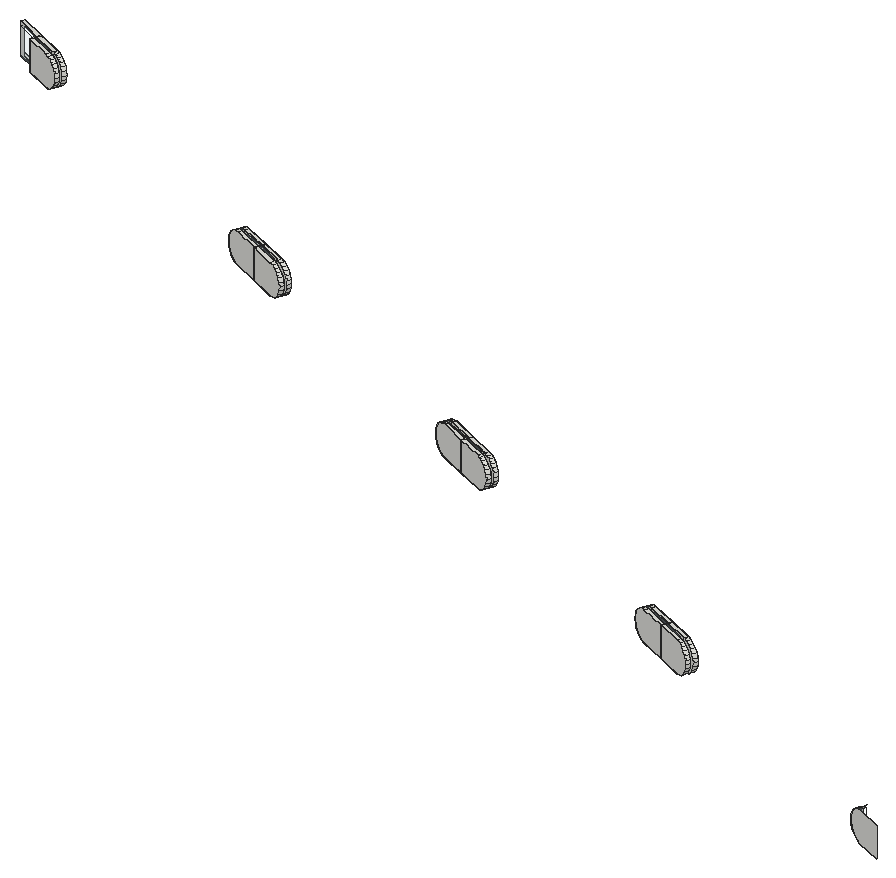
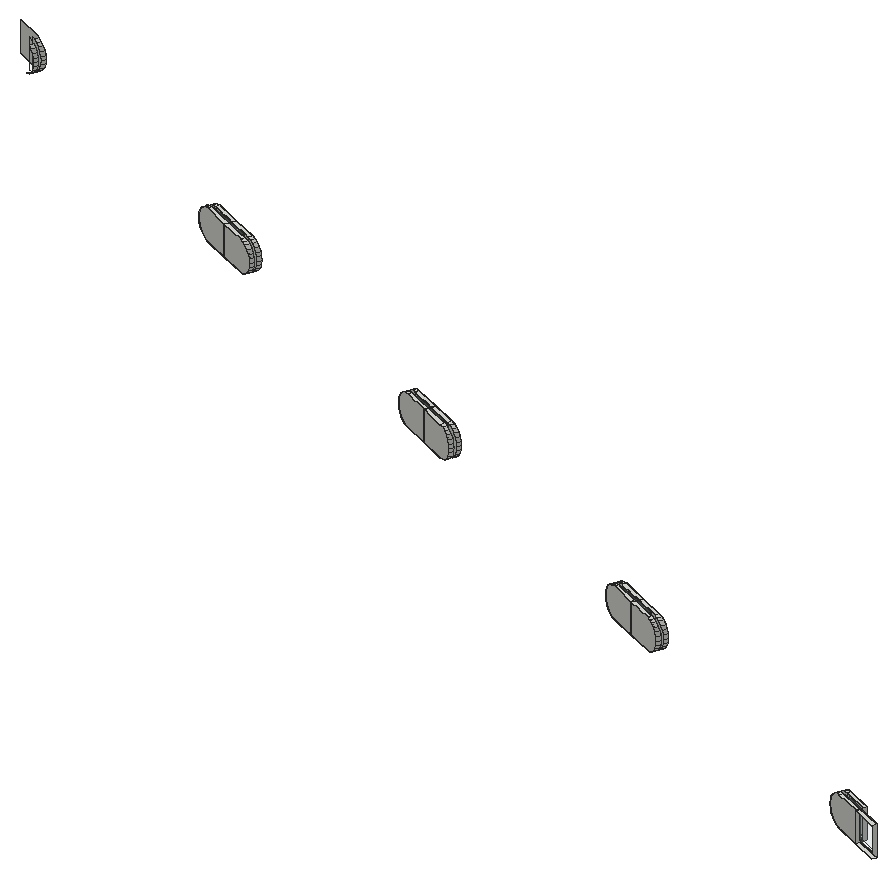
# SketchUp Ruby script. Lengths in inches.
U = 1.inch
M = Sketchup.active_model
def pt(a) = Geom::Point3d.new(a.map { |v| v * U })
def face(e, loops, mat)
  f = e.add_face(loops[0].map { |a| pt(a) })
  loops[1..].each { |l| e.add_face(l.map { |a| pt(a) }).erase! }
  f.material = f.back_material = mat if mat
  f
end
# faces: each face lists its corners as indices into pts; further lists are holes
def faces(e, pts, list, mat = nil) = list.each { |f| face(e, (f[0].is_a?(Array) ? f : [f]).map { |l| l.map { |i| pts[i] } }, mat) }
# xy, xz, yz: faces in a plane at the given z, y or x. An outline is a flat list of corners, or four numbers for a rectangle; further outlines are holes
def ring(l) = l.size == 4 ? [[l[0], l[1]], [l[2], l[1]], [l[2], l[3]], [l[0], l[3]]] : l.each_slice(2).to_a
def flat(e, list, mat, &to3) = list.each { |f| face(e, (f[0].is_a?(Array) ? f : [f]).map { |l| ring(l).map { |u, v| to3.(u, v) } }, mat) }
def xy(e, z, list, mat = nil) = flat(e, list, mat) { |x, y| [x, y, z] }
def xz(e, y, list, mat = nil) = flat(e, list, mat) { |x, z| [x, y, z] }
def yz(e, x, list, mat = nil) = flat(e, list, mat) { |y, z| [x, y, z] }
def lines(e, pts, list) = list.each { |a, b| e.add_line(pt(pts[a]), pt(pts[b])) }
# prism: a flat outline (further loops are holes) pulled along v
def prism(e, loops, v, mat = nil)
  f = face(e, loops, mat); d = Geom::Vector3d.new(v.map { |x| x * U })
  f.pushpull(f.normal.samedirection?(d) ? d.length : -d.length)
end
def box(e, o, s, mat = nil) = prism(e, [[o, [o[0] + s[0], o[1], o[2]], [o[0] + s[0], o[1] + s[1], o[2]], [o[0], o[1] + s[1], o[2]]]], [0, 0, s[2]], mat)
def at(x, y, z, deg = 0) = Geom::Transformation.translation(pt([x, y, z])) * Geom::Transformation.rotation(ORIGIN, Z_AXIS, deg.degrees)
def axes(o, x, y, z) = Geom::Transformation.new([*x, 0, *y, 0, *z, 0, *pt(o).to_a, 1])
def part(name) = M.definitions.add(name)
# library, detail: a bought-in or finely detailed component or shape, given as its bounding box
def library(name, o, s) = part(name).tap { |d| box(d.entities, o, s) }
def detail(e, o, s) = box(e.add_group.entities, o, s)
def put(e, d, t, mat = nil) = e.add_instance(d, t).tap { |i| i.material = mat if mat }
def group(e, t, mat = nil) = e.add_group.tap { |g| g.transformation = t; g.material = mat if mat }.entities
root = M.entities
M.materials.add("Glass_Safety_01").color = [204, 235, 244]
M.materials["Glass_Safety_01"].alpha = 0.1
xy(root,333,[[894.73,1068.32,892.93,1069.11,893.04,1069.36,894.71,1068.64,894.84,1068.58],[894.92,1068.76,894.79,1068.82,893.12,1069.54,893.23,1069.8,895.03,1069.01],[892.93,1069.11,891.125,1069.9,891.24,1070.15,893.04,1069.36],[893.12,1069.54,891.3125,1070.33,891.42,1070.58,893.23,1069.8],[872.89,1077.84,871.09,1078.625,871.2,1078.88,872.85,1078.16,873,1078.09],
  [873.08,1078.27,872.93,1078.34,871.27,1079.06,871.38,1079.31,873.19,1078.52],[871.09,1078.625,869.28,1079.41,869.39,1079.66,871.2,1078.88],[871.27,1079.06,869.47,1079.84,869.58,1080.1,871.38,1079.31],[850.22,1087.71,848.42,1088.5,848.53,1088.75,850.19,1088.03,850.33,1087.96],[850.41,1088.14,850.27,1088.21,848.61,1088.93,848.72,1089.18,850.52,1088.4],
  [848.42,1088.5,846.62,1089.28,846.73,1089.54,848.53,1088.75],[848.61,1088.93,846.8,1089.72,846.91,1089.97,848.72,1089.18],[825.64,1098.42,823.84,1099.2,823.95,1099.46,825.62,1098.73,825.75,1098.67],[825.83,1098.85,825.7,1098.91,824.02,1099.64,824.13,1099.89,825.94,1099.1],[824.02,1099.64,822.22,1100.42,822.33,1100.68,824.13,1099.89]])
xy(root,333.08,[[894.48,1068.73,893.04,1069.36,893.12,1069.54,894.5625,1068.92],[893.04,1069.36,891.6,1069.99,891.67,1070.17,893.12,1069.54],[872.64,1078.25,871.2,1078.88,871.27,1079.06,872.72,1078.43],[871.2,1078.88,869.75,1079.51,869.83,1079.6875,871.27,1079.06],[849.97,1088.12,848.53,1088.75,848.61,1088.93,850.05,1088.3],
  [848.53,1088.75,847.09,1089.38,847.16,1089.56,848.61,1088.93],[825.39,1098.83,823.95,1099.46,824.02,1099.64,825.47,1099.01],[823.95,1099.46,822.5,1100.08,822.58,1100.27,824.02,1099.64]],"Glass_Safety_01")
xy(root,335.05,[[894.48,1068.73,894.5625,1068.92,893.12,1069.54,893.04,1069.36],[893.04,1069.36,893.12,1069.54,891.67,1070.17,891.6,1069.99],[872.64,1078.25,872.72,1078.43,871.27,1079.06,871.2,1078.88],[871.2,1078.88,871.27,1079.06,869.83,1079.6875,869.75,1079.51],[849.97,1088.12,850.05,1088.3,848.61,1088.93,848.53,1088.75],
  [848.53,1088.75,848.61,1088.93,847.16,1089.56,847.09,1089.38],[825.39,1098.83,825.47,1099.01,824.02,1099.64,823.95,1099.46],[823.95,1099.46,824.02,1099.64,822.58,1100.27,822.5,1100.08]],"Glass_Safety_01")
xy(root,335.125,[[894.73,1068.32,894.84,1068.58,894.71,1068.64,893.04,1069.36,892.93,1069.11],[894.92,1068.76,895.03,1069.01,893.23,1069.8,893.12,1069.54,894.79,1068.82],[892.93,1069.11,893.04,1069.36,891.24,1070.15,891.125,1069.9],[893.12,1069.54,893.23,1069.8,891.42,1070.58,891.3125,1070.33],[872.89,1077.84,873,1078.09,872.85,1078.16,871.2,1078.88,871.09,1078.625],
  [873.08,1078.27,873.19,1078.52,871.38,1079.31,871.27,1079.06,872.93,1078.34],[871.09,1078.625,871.2,1078.88,869.39,1079.66,869.28,1079.41],[871.27,1079.06,871.38,1079.31,869.58,1080.1,869.47,1079.84],[850.22,1087.71,850.33,1087.96,850.19,1088.03,848.53,1088.75,848.42,1088.5],[850.41,1088.14,850.52,1088.4,848.72,1089.18,848.61,1088.93,850.27,1088.21],
  [848.42,1088.5,848.53,1088.75,846.73,1089.54,846.62,1089.28],[848.61,1088.93,848.72,1089.18,846.91,1089.97,846.8,1089.72],[825.64,1098.42,825.75,1098.67,825.62,1098.73,823.95,1099.46,823.84,1099.2],[825.83,1098.85,825.94,1099.1,824.13,1099.89,824.02,1099.64,825.7,1098.91],[824.02,1099.64,824.13,1099.89,822.33,1100.68,822.22,1100.42]])
p = [[916.56,1058.82,335.125],[914.75,1059.61,335.125],[914.5,1059.72,335.09],[914.27,1059.82,334.98],[914.06,1059.91,334.8125],[913.91,1059.97,334.59],
  [913.8125,1060.02,334.34],[913.78,1060.03,334.0625],[913.8125,1060.02,333.79],[913.91,1059.97,333.53],[914.06,1059.91,333.3125],[914.27,1059.82,333.14],
  [914.5,1059.72,333.04],[914.75,1059.61,333],[916.56,1058.82,333],[914.375,1060.07,333.14],[914.61,1059.97,333.04],[914.86,1059.86,333],
  [914.86,1059.86,335.125],[914.61,1059.97,335.09],[914.375,1060.07,334.98],[914.17,1060.16,334.8125],[914.02,1060.23,334.59],[913.92,1060.27,334.34],
  [913.89,1060.28,334.0625],[913.92,1060.27,333.79],[914.02,1060.23,333.53],[914.17,1060.16,333.3125],[914.94,1060.04,335.125],[914.94,1060.04,333],
  [914.69,1060.15,333.04],[914.46,1060.25,333.14],[914.25,1060.34,333.3125],[914.1,1060.41,333.53],[914,1060.45,333.79],[913.97,1060.46,334.0625],
  [914,1060.45,334.34],[914.1,1060.41,334.59],[914.25,1060.34,334.8125],[914.46,1060.25,334.98],[914.69,1060.15,335.09],[914.57,1060.5,333.14],
  [914.8,1060.4,333.04],[894.73,1068.32,335.125],[892.93,1069.11,335.125],[892.93,1069.11,333],[894.73,1068.32,333],[894.99,1068.22,333.04],
  [895.22,1068.11,333.14],[895.42,1068.02,333.3125],[895.58,1067.96,333.53],[895.68,1067.91,333.79],[895.71,1067.9,334.0625],[895.68,1067.91,334.34],
  [895.58,1067.96,334.59],[895.42,1068.02,334.8125],[895.22,1068.11,334.98],[894.99,1068.22,335.09],[895.1,1068.47,333.04],[895.33,1068.37,333.14],
  [894.84,1068.58,333],[894.71,1068.64,333],[894.71,1068.64,335.125],[894.84,1068.58,335.125],[895.1,1068.47,335.09],[895.33,1068.37,334.98],
  [895.53,1068.28,334.8125],[895.6875,1068.21,334.59],[895.79,1068.17,334.34],[895.82,1068.15,334.0625],[895.79,1068.17,333.79],[895.6875,1068.21,333.53],
  [895.53,1068.28,333.3125],[894.92,1068.76,335.125],[894.79,1068.82,335.125],[894.79,1068.82,333],[894.92,1068.76,333],[895.18,1068.65,333.04],
  [895.41,1068.55,333.14],[895.61,1068.46,333.3125],[895.77,1068.39,333.53],[895.86,1068.35,333.79],[895.9,1068.33,334.0625],[895.86,1068.35,334.34],
  [895.77,1068.39,334.59],[895.61,1068.46,334.8125],[895.41,1068.55,334.98],[895.18,1068.65,335.09],[895.29,1068.9,333.04],[895.52,1068.8,333.14],
  [893.04,1069.36,335.125],[893.04,1069.36,333],[893.04,1069.36,333.08],[894.48,1068.73,333.08],[894.48,1068.73,335.05],[893.04,1069.36,335.05],
  [893.23,1069.8,335.125],[895.03,1069.01,335.125],[895.29,1068.9,335.09],[895.52,1068.8,334.98],[895.72,1068.71,334.8125],[895.88,1068.64,334.59],
  [895.97,1068.6,334.34],[896.01,1068.59,334.0625],[895.97,1068.6,333.79],[895.88,1068.64,333.53],[895.72,1068.71,333.3125],[895.03,1069.01,333],
  [893.23,1069.8,333],[893.12,1069.54,333],[893.12,1069.54,335.125],[893.12,1069.54,335.05],[894.5625,1068.92,335.05],[894.5625,1068.92,333.08],
  [893.12,1069.54,333.08],[891.125,1069.9,335.125],[890.87,1070.01,335.09],[890.64,1070.11,334.98],[890.4375,1070.2,334.8125],[890.28,1070.26,334.59],
  [890.18,1070.31,334.34],[890.15,1070.32,334.0625],[890.18,1070.31,333.79],[890.28,1070.26,333.53],[890.4375,1070.2,333.3125],[890.64,1070.11,333.14],
  [890.87,1070.01,333.04],[891.125,1069.9,333],[891.24,1070.15,333],[891.24,1070.15,335.125],[891.6,1069.99,335.05],[891.6,1069.99,333.08],
  [891.3125,1070.33,335.125],[891.3125,1070.33,333],[891.67,1070.17,333.08],[891.67,1070.17,335.05],[891.42,1070.58,335.125],[891.42,1070.58,333],
  [891.17,1070.69,333.04],[890.9375,1070.79,333.14],[890.73,1070.88,333.3125],[890.58,1070.95,333.53],[890.48,1070.99,333.79],[890.45,1071.01,334.0625],
  [890.48,1070.99,334.34],[890.58,1070.95,334.59],[890.73,1070.88,334.8125],[890.9375,1070.79,334.98],[891.17,1070.69,335.09],[890.98,1070.26,333.04],
  [890.75,1070.36,333.14],[890.98,1070.26,335.09],[890.75,1070.36,334.98],[890.55,1070.45,334.8125],[890.39,1070.52,334.59],[890.29,1070.56,334.34],
  [890.26,1070.57,334.0625],[890.29,1070.56,333.79],[890.39,1070.52,333.53],[890.55,1070.45,333.3125],[891.0625,1070.44,333.04],[890.83,1070.54,333.14],
  [890.625,1070.63,333.3125],[890.47,1070.7,333.53],[890.37,1070.74,333.79],[890.34,1070.75,334.0625],[890.37,1070.74,334.34],[890.47,1070.7,334.59],
  [890.625,1070.63,334.8125],[890.83,1070.54,334.98],[891.0625,1070.44,335.09],[872.89,1077.84,335.125],[871.09,1078.625,335.125],[871.09,1078.625,333],
  [872.89,1077.84,333],[873.14,1077.73,333.04],[873.38,1077.625,333.14],[873.58,1077.54,333.3125],[873.73,1077.47,333.53],[873.83,1077.43,333.79],
  [873.87,1077.41,334.0625],[873.83,1077.43,334.34],[873.73,1077.47,334.59],[873.58,1077.54,334.8125],[873.38,1077.625,334.98],[873.14,1077.73,335.09],
  [873.25,1077.98,333.04],[873.49,1077.88,333.14],[873,1078.09,333],[872.85,1078.16,333],[872.85,1078.16,335.125],[873,1078.09,335.125],
  [873.25,1077.98,335.09],[873.49,1077.88,334.98],[873.69,1077.79,334.8125],[873.84,1077.72,334.59],[873.94,1077.68,334.34],[873.98,1077.67,334.0625],
  [873.94,1077.68,333.79],[873.84,1077.72,333.53],[873.69,1077.79,333.3125],[873.08,1078.27,335.125],[872.93,1078.34,335.125],[872.93,1078.34,333],
  [873.08,1078.27,333],[873.33,1078.16,333.04],[873.57,1078.06,333.14],[873.77,1077.97,333.3125],[873.92,1077.9,333.53],[874.02,1077.86,333.79],
  [874.05,1077.85,334.0625],[874.02,1077.86,334.34],[873.92,1077.9,334.59],[873.77,1077.97,334.8125],[873.57,1078.06,334.98],[873.33,1078.16,335.09],
  [871.38,1079.31,335.125],[873.19,1078.52,335.125],[873.44,1078.41,335.09],[873.68,1078.3125,334.98],[873.88,1078.22,334.8125],[874.03,1078.16,334.59],
  [874.13,1078.11,334.34],[874.16,1078.1,334.0625],[874.13,1078.11,333.79],[874.03,1078.16,333.53],[873.88,1078.22,333.3125],[873.68,1078.3125,333.14],
  [873.44,1078.41,333.04],[873.19,1078.52,333],[871.38,1079.31,333],[871.2,1078.88,335.125],[871.2,1078.88,333],[871.2,1078.88,333.08],
  [872.64,1078.25,333.08],[872.64,1078.25,335.05],[871.2,1078.88,335.05],[871.27,1079.06,333],[871.27,1079.06,335.125],[871.27,1079.06,335.05],
  [872.72,1078.43,335.05],[872.72,1078.43,333.08],[871.27,1079.06,333.08],[869.28,1079.41,335.125],[869.03,1079.52,335.09],[868.79,1079.62,334.98],
  [868.59,1079.71,334.8125],[868.4375,1079.78,334.59],[868.34,1079.82,334.34],[868.31,1079.84,334.0625],[868.34,1079.82,333.79],[868.4375,1079.78,333.53],
  [868.59,1079.71,333.3125],[868.79,1079.62,333.14],[869.03,1079.52,333.04],[869.28,1079.41,333],[869.39,1079.66,333],[869.39,1079.66,335.125],
  [869.75,1079.51,335.05],[869.75,1079.51,333.08],[869.47,1079.84,335.125],[869.47,1079.84,333],[869.83,1079.6875,333.08],[869.83,1079.6875,335.05],
  [869.58,1080.1,335.125],[869.58,1080.1,333],[869.33,1080.21,333.04],[869.09,1080.31,333.14],[868.89,1080.4,333.3125],[868.74,1080.46,333.53],
  [868.64,1080.51,333.79],[868.61,1080.52,334.0625],[868.64,1080.51,334.34],[868.74,1080.46,334.59],[868.89,1080.4,334.8125],[869.09,1080.31,334.98],
  [869.33,1080.21,335.09],[869.14,1079.77,333.04],[868.9,1079.875,333.14],[869.14,1079.77,335.09],[868.9,1079.875,334.98],[868.7,1079.96,334.8125],
  [868.55,1080.03,334.59],[868.45,1080.07,334.34],[868.42,1080.09,334.0625],[868.45,1080.07,333.79],[868.55,1080.03,333.53],[868.7,1079.96,333.3125],
  [869.22,1079.95,333.04],[868.98,1080.06,333.14],[868.78,1080.14,333.3125],[868.625,1080.21,333.53],[868.53,1080.25,333.79],[868.5,1080.27,334.0625],
  [868.53,1080.25,334.34],[868.625,1080.21,334.59],[868.78,1080.14,334.8125],[868.98,1080.06,334.98],[869.22,1079.95,335.09],[850.22,1087.71,335.125],
  [848.42,1088.5,335.125],[848.42,1088.5,333],[850.22,1087.71,333],[850.48,1087.6,333.04],[850.71,1087.5,333.14],[850.91,1087.41,333.3125],
  [851.07,1087.34,333.53],[851.17,1087.3,333.79],[851.2,1087.29,334.0625],[851.17,1087.3,334.34],[851.07,1087.34,334.59],[850.91,1087.41,334.8125],
  [850.71,1087.5,334.98],[850.48,1087.6,335.09],[850.33,1087.96,333],[850.19,1088.03,333],[850.19,1088.03,335.125],[850.33,1087.96,335.125],
  [850.59,1087.85,335.09],[850.82,1087.75,334.98],[851.02,1087.66,334.8125],[851.18,1087.6,334.59],[851.28,1087.55,334.34],[851.31,1087.54,334.0625],
  [851.28,1087.55,333.79],[851.18,1087.6,333.53],[851.02,1087.66,333.3125],[850.82,1087.75,333.14],[850.59,1087.85,333.04],[850.41,1088.14,335.125],
  [850.27,1088.21,335.125],[850.27,1088.21,333],[850.41,1088.14,333],[850.67,1088.03,333.04],[850.9,1087.93,333.14],[851.1,1087.84,333.3125],
  [851.26,1087.78,333.53],[851.35,1087.73,333.79],[851.39,1087.72,334.0625],[851.35,1087.73,334.34],[851.26,1087.78,334.59],[851.1,1087.84,334.8125],
  [850.9,1087.93,334.98],[850.67,1088.03,335.09],[850.78,1088.29,333.04],[851.01,1088.18,333.14],[848.53,1088.75,335.125],[848.53,1088.75,333],
  [848.53,1088.75,333.08],[849.97,1088.12,333.08],[849.97,1088.12,335.05],[848.53,1088.75,335.05],[848.72,1089.18,335.125],[850.52,1088.4,335.125],
  [850.78,1088.29,335.09],[851.01,1088.18,334.98],[851.21,1088.1,334.8125],[851.37,1088.03,334.59],[851.46,1087.99,334.34],[851.5,1087.97,334.0625],
  [851.46,1087.99,333.79],[851.37,1088.03,333.53],[851.21,1088.1,333.3125],[850.52,1088.4,333],[848.72,1089.18,333],[848.61,1088.93,333],
  [848.61,1088.93,335.125],[848.61,1088.93,335.05],[850.05,1088.3,335.05],[850.05,1088.3,333.08],[848.61,1088.93,333.08],[846.62,1089.28,335.125],
  [846.36,1089.39,335.09],[846.13,1089.49,334.98],[845.93,1089.58,334.8125],[845.77,1089.65,334.59],[845.67,1089.69,334.34],[845.64,1089.71,334.0625],
  [845.67,1089.69,333.79],[845.77,1089.65,333.53],[845.93,1089.58,333.3125],[846.13,1089.49,333.14],[846.36,1089.39,333.04],[846.62,1089.28,333],
  [846.73,1089.54,333],[846.73,1089.54,335.125],[847.09,1089.38,335.05],[847.09,1089.38,333.08],[846.8,1089.72,335.125],[846.8,1089.72,333],
  [847.16,1089.56,333.08],[847.16,1089.56,335.05],[846.91,1089.97,335.125],[846.91,1089.97,333],[846.66,1090.08,333.04],[846.43,1090.18,333.14],
  [846.22,1090.27,333.3125],[846.07,1090.34,333.53],[845.97,1090.38,333.79],[845.9375,1090.39,334.0625],[845.97,1090.38,334.34],[846.07,1090.34,334.59],
  [846.22,1090.27,334.8125],[846.43,1090.18,334.98],[846.66,1090.08,335.09],[846.47,1089.64,333.04],[846.24,1089.75,333.14],[846.47,1089.64,335.09],
  [846.24,1089.75,334.98],[846.04,1089.84,334.8125],[845.88,1089.9,334.59],[845.78,1089.95,334.34],[845.75,1089.96,334.0625],[845.78,1089.95,333.79],
  [845.88,1089.9,333.53],[846.04,1089.84,333.3125],[846.55,1089.83,333.04],[846.32,1089.93,333.14],[846.11,1090.02,333.3125],[845.96,1090.08,333.53],
  [845.86,1090.125,333.79],[845.83,1090.14,334.0625],[845.86,1090.125,334.34],[845.96,1090.08,334.59],[846.11,1090.02,334.8125],[846.32,1089.93,334.98],
  [846.55,1089.83,335.09],[825.64,1098.42,335.125],[823.84,1099.2,335.125],[823.84,1099.2,333],[825.64,1098.42,333],[825.89,1098.31,333.04],
  [826.13,1098.21,333.14],[826.33,1098.12,333.3125],[826.48,1098.05,333.53],[826.58,1098.01,333.79],[826.62,1097.99,334.0625],[826.58,1098.01,334.34],
  [826.48,1098.05,334.59],[826.33,1098.12,334.8125],[826.13,1098.21,334.98],[825.89,1098.31,335.09],[825.75,1098.67,333],[825.62,1098.73,333],
  [825.62,1098.73,335.125],[825.75,1098.67,335.125],[826,1098.56,335.09],[826.24,1098.46,334.98],[826.44,1098.37,334.8125],[826.59,1098.3,334.59],
  [826.69,1098.26,334.34],[826.73,1098.25,334.0625],[826.69,1098.26,333.79],[826.59,1098.3,333.53],[826.44,1098.37,333.3125],[826.24,1098.46,333.14],
  [826,1098.56,333.04],[825.83,1098.85,335.125],[825.7,1098.91,335.125],[825.7,1098.91,333],[825.83,1098.85,333],[826.08,1098.74,333.04],
  [826.32,1098.64,333.14],[826.52,1098.55,333.3125],[826.67,1098.48,333.53],[826.77,1098.44,333.79],[826.8,1098.43,334.0625],[826.77,1098.44,334.34],
  [826.67,1098.48,334.59],[826.52,1098.55,334.8125],[826.32,1098.64,334.98],[826.08,1098.74,335.09],[826.19,1098.99,333.04],[826.43,1098.89,333.14],
  [823.95,1099.46,335.125],[823.95,1099.46,333],[823.95,1099.46,333.08],[825.39,1098.83,333.08],[825.39,1098.83,335.05],[823.95,1099.46,335.05],
  [824.13,1099.89,335.125],[825.94,1099.1,335.125],[826.19,1098.99,335.09],[826.43,1098.89,334.98],[826.63,1098.8,334.8125],[826.78,1098.74,334.59],
  [826.88,1098.69,334.34],[826.91,1098.68,334.0625],[826.88,1098.69,333.79],[826.78,1098.74,333.53],[826.63,1098.8,333.3125],[825.94,1099.1,333],
  [824.13,1099.89,333],[824.02,1099.64,333],[824.02,1099.64,335.125],[824.02,1099.64,335.05],[825.47,1099.01,335.05],[825.47,1099.01,333.08],
  [824.02,1099.64,333.08],[822.22,1100.42,335.125],[822.22,1100.42,333],[822.58,1100.27,333.08],[822.58,1100.27,335.05],[914.36,1060.59,333.3125],
  [822.5,1100.08,333.08],[822.5,1100.08,335.05],[914.21,1060.66,333.53],[914.11,1060.7,333.79],[914.08,1060.72,334.0625],[914.11,1060.7,334.34],
  [914.21,1060.66,334.59],[914.36,1060.59,334.8125],[914.57,1060.5,334.98]]
faces(root,p,[[0,1,2,3,4,5,6,7,8,9,10,11,12,13,14],[15,16,12,11],[30,31,41,42],[43,44,45,46,47,48,49,50,51,52,53,54,55,56,57],[58,59,48,47],[60,58,47,46],[60,61,62,63,64,65,66,67,68,69,70,71,72,59,58],[73,74,75,76,77,78,79,80,81,82,83,84,85,86,87],
  [78,77,88,89],[90,62,61,91,92,93,94,95],[96,97,98,99,100,101,102,103,104,105,106,89,88,107,108],[77,76,107,88],[109,75,74,110,111,112,113,114],[44,115,116,117,118,119,120,121,122,123,124,125,126,127,45],[92,91,45,44,90,95],[91,128,129,90,95,130,131,92],
  [110,132,133,109,114,134,135,111],[109,114,111,110,96,108],[136,96,108,137,138,139,140,141,142,143,144,145,146,147,148],[149,128,127,126],[150,149,126,125],[133,160,138,137],[160,161,139,138],[171,172,173,174,175,176,177,178,179,180,181,182,183,184,185],
  [186,187,176,175],[188,186,175,174],[188,189,190,191,192,193,194,195,196,197,198,199,200,187,186],[201,202,203,204,205,206,207,208,209,210,211,212,213,214,215],[216,217,218,219,220,221,222,223,224,225,226,227,228,229,230],[206,205,228,227],[231,190,189,232,233,234,235,236],[205,204,229,228],
  [237,203,202,238,239,240,241,242],[172,243,244,245,246,247,248,249,250,251,252,253,254,255,173],[233,232,173,172,231,236],[232,256,257,231,236,258,259,233],[238,260,261,237,242,262,263,239],[237,242,239,238,216,230],[264,216,230,265,266,267,268,269,270,271,272,273,274,275,276],[277,256,255,254],
  [278,277,254,253],[261,288,266,265],[288,289,267,266],[299,300,301,302,303,304,305,306,307,308,309,310,311,312,313],[314,315,316,317,318,319,320,321,322,323,324,325,326,327,328],[328,327,304,303],[314,328,303,302],[329,330,331,332,333,334,335,336,337,338,339,340,341,342,343],
  [334,333,344,345],[346,316,315,347,348,349,350,351],[352,353,354,355,356,357,358,359,360,361,362,345,344,363,364],[333,332,363,344],[365,331,330,366,367,368,369,370],[300,371,372,373,374,375,376,377,378,379,380,381,382,383,301],[348,347,301,300,346,351],[347,384,385,346,351,386,387,348],
  [366,388,389,365,370,390,391,367],[365,370,367,366,352,364],[392,352,364,393,394,395,396,397,398,399,400,401,402,403,404],[405,384,383,382],[406,405,382,381],[389,416,394,393],[416,417,395,394],[427,428,429,430,431,432,433,434,435,436,437,438,439,440,441],
  [442,443,444,445,446,447,448,449,450,451,452,453,454,455,456],[456,455,432,431],[442,456,431,430],[457,458,459,460,461,462,463,464,465,466,467,468,469,470,471],[462,461,472,473],[474,444,443,475,476,477,478,479],[480,481,482,483,484,485,486,487,488,489,490,473,472,491,492],[461,460,491,472],
  [493,459,458,494,495,496,497,498],[476,475,429,428,474,479],[494,499,500,493,498,501,502,495],[493,498,495,494,480,492],[27,15,11,10],[31,32,503,41],[59,72,49,48],[79,78,89,106],
  [159,150,125,124],[161,162,140,139],[187,200,177,176],[207,206,227,226],[287,278,253,252],[289,290,268,267],[327,326,305,304],[335,334,345,362],
  [415,406,381,380],[417,418,396,395],[455,454,433,432],[463,462,473,490],[26,27,10,9],[32,33,506,503],[72,71,50,49],[80,79,106,105],
  [158,159,124,123],[162,163,141,140],[200,199,178,177],[208,207,226,225],[286,287,252,251],[290,291,269,268],[326,325,306,305],[336,335,362,361],
  [414,415,380,379],[418,419,397,396],[454,453,434,433],[464,463,490,489],[25,26,9,8],[33,34,507,506],[71,70,51,50],[81,80,105,104],
  [157,158,123,122],[163,164,142,141],[199,198,179,178],[209,208,225,224],[285,286,251,250],[291,292,270,269],[325,324,307,306],[337,336,361,360],
  [413,414,379,378],[419,420,398,397],[453,452,435,434],[465,464,489,488],[24,25,8,7],[34,35,508,507],[70,69,52,51],[82,81,104,103],
  [156,157,122,121],[164,165,143,142],[198,197,180,179],[210,209,224,223],[284,285,250,249],[292,293,271,270],[324,323,308,307],[338,337,360,359],
  [412,413,378,377],[420,421,399,398],[452,451,436,435],[466,465,488,487],[23,24,7,6],[35,36,509,508],[69,68,53,52],[83,82,103,102],
  [155,156,121,120],[165,166,144,143],[197,196,181,180],[211,210,223,222],[283,284,249,248],[293,294,272,271],[323,322,309,308],[339,338,359,358],
  [411,412,377,376],[421,422,400,399],[451,450,437,436],[467,466,487,486],[22,23,6,5],[36,37,510,509],[68,67,54,53],[84,83,102,101],
  [154,155,120,119],[166,167,145,144],[196,195,182,181],[212,211,222,221],[282,283,248,247],[294,295,273,272],[322,321,310,309],[340,339,358,357],
  [410,411,376,375],[422,423,401,400],[450,449,438,437],[468,467,486,485],[21,22,5,4],[37,38,511,510],[67,66,55,54],[85,84,101,100],
  [153,154,119,118],[167,168,146,145],[195,194,183,182],[213,212,221,220],[281,282,247,246],[295,296,274,273],[321,320,311,310],[341,340,357,356],
  [409,410,375,374],[423,424,402,401],[449,448,439,438],[469,468,485,484],[20,21,4,3],[38,39,512,511],[66,65,56,55],[86,85,100,99],
  [152,153,118,117],[168,169,147,146],[194,193,184,183],[214,213,220,219],[280,281,246,245],[296,297,275,274],[320,319,312,311],[342,341,356,355],
  [408,409,374,373],[424,425,403,402],[448,447,440,439],[470,469,484,483],[19,20,3,2],[65,64,57,56],[87,86,99,98],[151,152,117,116],
  [169,170,148,147],[193,192,185,184],[215,214,219,218],[279,280,245,244],[297,298,276,275],[319,318,313,312],[343,342,355,354],[407,408,373,372],
  [425,426,404,403],[447,446,441,440],[471,470,483,482],[64,63,43,57],[73,87,98,97],[129,151,116,115],[170,132,136,148],[192,191,171,185],
  [201,215,218,217],[257,279,244,243],[298,260,264,276],[318,317,299,313],[329,343,354,353],[385,407,372,371],[426,388,392,404],[446,445,427,441],
  [457,471,482,481]])
faces(root,p,[[17,18,19,20,21,22,23,24,25,26,27,15,16],[28,29,30,31,32,33,34,35,36,37,38,39,40],[128,129,151,152,153,154,155,156,157,158,159,150,149],[132,133,160,161,162,163,164,165,166,167,168,169,170],[256,257,279,280,281,282,283,284,285,286,287,278,277],[260,261,288,289,290,291,292,293,294,295,296,297,298],[384,385,407,408,409,410,411,412,413,414,415,406,405],[388,389,416,417,418,419,420,421,422,423,424,425,426],
  [93,92,95,94],[113,112,94,93],[114,113,112,111],[92,131,130,95],[114,92,95,111],[134,114,111,135],[131,130,135,134],[234,233,236,235],
  [241,240,235,234],[242,241,240,239],[233,259,258,236],[242,233,236,239],[262,242,239,263],[259,258,263,262],[349,348,351,350],[369,368,350,349],
  [370,369,368,367],[348,387,386,351],[370,348,351,367],[390,370,367,391],[387,386,391,390],[477,476,479,478],[497,496,478,477],[498,497,496,495],
  [476,504,505,479],[498,476,479,495],[501,498,495,502]],"Glass_Safety_01")
